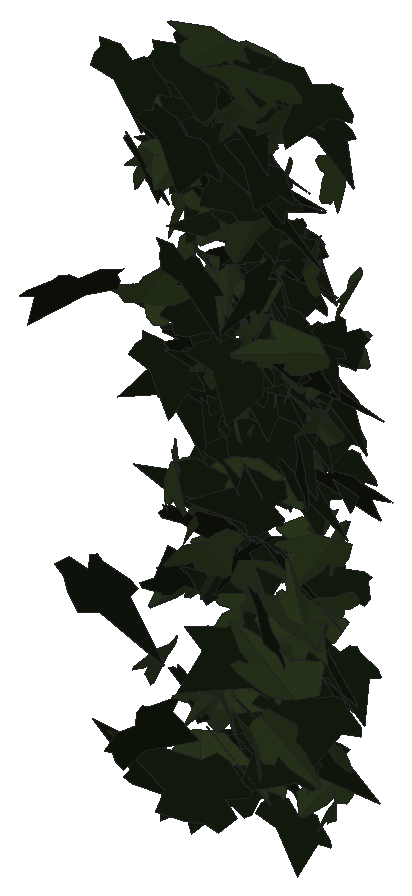
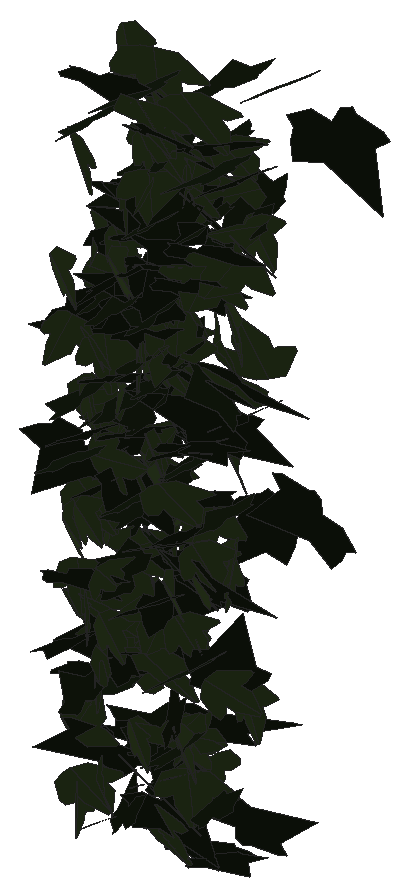
# SketchUp Ruby script. Lengths in millimetres.
U = 1.mm
M = Sketchup.active_model
def pt(a) = Geom::Point3d.new(a.map { |v| v * U })
def face(e, loops, mat)
  f = e.add_face(loops[0].map { |a| pt(a) })
  loops[1..].each { |l| e.add_face(l.map { |a| pt(a) }).erase! }
  f.material = f.back_material = mat if mat
  f
end
# faces: each face lists its corners as indices into pts; further lists are holes
def faces(e, pts, list, mat = nil) = list.each { |f| face(e, (f[0].is_a?(Array) ? f : [f]).map { |l| l.map { |i| pts[i] } }, mat) }
# xy, xz, yz: faces in a plane at the given z, y or x. An outline is a flat list of corners, or four numbers for a rectangle; further outlines are holes
def ring(l) = l.size == 4 ? [[l[0], l[1]], [l[2], l[1]], [l[2], l[3]], [l[0], l[3]]] : l.each_slice(2).to_a
def flat(e, list, mat, &to3) = list.each { |f| face(e, (f[0].is_a?(Array) ? f : [f]).map { |l| ring(l).map { |u, v| to3.(u, v) } }, mat) }
def xy(e, z, list, mat = nil) = flat(e, list, mat) { |x, y| [x, y, z] }
def xz(e, y, list, mat = nil) = flat(e, list, mat) { |x, z| [x, y, z] }
def yz(e, x, list, mat = nil) = flat(e, list, mat) { |y, z| [x, y, z] }
def lines(e, pts, list) = list.each { |a, b| e.add_line(pt(pts[a]), pt(pts[b])) }
# prism: a flat outline (further loops are holes) pulled along v
def prism(e, loops, v, mat = nil)
  f = face(e, loops, mat); d = Geom::Vector3d.new(v.map { |x| x * U })
  f.pushpull(f.normal.samedirection?(d) ? d.length : -d.length)
end
def box(e, o, s, mat = nil) = prism(e, [[o, [o[0] + s[0], o[1], o[2]], [o[0] + s[0], o[1] + s[1], o[2]], [o[0], o[1] + s[1], o[2]]]], [0, 0, s[2]], mat)
def at(x, y, z, deg = 0) = Geom::Transformation.translation(pt([x, y, z])) * Geom::Transformation.rotation(ORIGIN, Z_AXIS, deg.degrees)
def axes(o, x, y, z) = Geom::Transformation.new([*x, 0, *y, 0, *z, 0, *pt(o).to_a, 1])
def part(name) = M.definitions.add(name)
# library, detail: a bought-in or finely detailed component or shape, given as its bounding box
def library(name, o, s) = part(name).tap { |d| box(d.entities, o, s) }
def detail(e, o, s) = box(e.add_group.entities, o, s)
def put(e, d, t, mat = nil) = e.add_instance(d, t).tap { |i| i.material = mat if mat }
def group(e, t, mat = nil) = e.add_group.tap { |g| g.transformation = t; g.material = mat if mat }.entities
root = M.entities
M.materials.add("efeu1").color = [18, 25, 13]
M.materials.add("efeu2").color = [43, 57, 29]
c1 = part("ivyleaf_10")
p = [[0,12.8,-0.8],[-1.5,51.3,-10.9],[-4.9,51,-11.6],[-13.6,26.5,-7.3],[-13.2,15.9,-4.6],[-21.1,19.3,-7.2],
  [-29.5,16.3,-8.3],[-29.2,8.3,-6.2],[-19.7,-9.8,0.5],[-7.6,-13,4],[1,-12.2,5.8],[-0.4,51.1,-11.1],
  [-1.5,51.1,-10.9],[1,-12.4,5.9],[16.9,-12.4,3.5],[35.1,9.1,-5.1],[35,12.9,-6.1],[20.5,16.4,-4.9],
  [15.8,15,-3.8],[15.3,27.6,-7.1],[12.8,31.3,-7.8]]
faces(c1.entities,p,[[0,1,2,3,4,5,6,7,8,9,10],[11,12,0,13,14,15,16,17,18,19,20]],"efeu2")
c2 = part("ivyleaf_9")
p = [[39.1,54.8,31.7],[34.5,51.8,30.2],[-5.3,25.2,17.3],[-17.9,28.3,20.9],[-21.6,21.7,17],[-20.2,4.3,5.3],
  [-22.9,-0.3,2.5],[-17.1,-4,-0.6],[-2,-2.1,-1.2],[-0.7,-15.4,-10.1],[16.6,-22.3,-16.7],[21.1,-15.1,-12.5],
  [32.7,-10.7,-11],[46.1,-1.8,-6.6],[30.8,11.2,3.8]]
faces(c2.entities,p,[[0,1,2,3,4,5,6,7,8,9,10,11,12,13,14]],"efeu1")
put(root,c1,axes([2370.1,876.6,2356.8],[0.60294,-0.8909,-0.24909],[-0.05038,0.25445,-0.94375],[1.75987,0.31251,0.05832]))
put(root,c1,axes([2378.9,889.4,1882.8],[-0.34168,-0.62629,0.72512],[-0.30507,-0.70771,-0.65094],[1.79784,-0.23911,0.02736]))
put(root,c1,axes([2372.9,830.5,2450.6],[-0.06453,-0.98735,0.19467],[0.00299,-0.19483,-0.9879],[1.9153,-0.03296,0.0081]))
put(root,c1,axes([2354.5,855.3,2466.6],[0.48026,0.03585,-1.00007],[0.86211,0.91557,0.14712],[1.69827,-0.47492,0.20813]))
put(root,c1,axes([2363.1,882.7,2430.9],[-1.63571,-0.35297,-0.36931],[0.67826,0.10361,-0.92839],[0.69661,-0.92969,0.03675]))
put(root,c2,axes([2408.1,817,1664.1],[0.1409,-0.06142,0.97578],[-1.59712,0.49814,0.09503],[-0.95482,-0.8423,-0.01495]))
put(root,c1,axes([2390.6,853.3,2039.9],[-0.88376,0.56277,0.68264],[-0.77206,0.54969,-0.72911],[-1.49633,-0.616,-0.02698]))
put(root,c1,axes([2373,822.3,2270.3],[-1.0554,-0.86595,0.15564],[0.17943,0.12443,1.02822],[-1.66484,0.56237,0.01215]))
put(root,c2,axes([2363.9,893.8,2108.3],[0.13845,-0.89281,0.30246],[0.11131,-0.2985,-0.89519],[1.7906,0.08759,0.03226]))
put(root,c1,axes([2385.4,858.4,2023.6],[0.17024,-0.72433,-0.6179],[0.02917,0.62164,-0.72649],[1.81176,0.05805,0.06976]))
put(root,c2,axes([2381.9,870.7,1884],[1.11058,0.35379,0.7817],[-1.27053,-0.40669,0.68241],[1.0259,-0.88666,-0.00109]))
put(root,c2,axes([2423,854.5,2254.5],[-1.28585,0.28963,0.67405],[-1.2505,0.16875,-0.73109],[-0.62112,-0.93933,0.07649]))
put(root,c2,axes([2375.3,903.8,1728.1],[-0.29406,-0.50177,0.73344],[0.1244,-0.74884,-0.49854],[1.68671,-0.03225,0.16464]))
put(root,c2,axes([2379.1,873.8,2522.8],[-0.482,-1.00816,0.31724],[-0.09348,-0.31464,-1.03912],[2.00932,-0.25648,0.02776]))
put(root,c2,axes([2397,899.2,2443],[-1.52442,-0.55514,-0.05475],[0.07746,0.03739,-0.97452],[1.05883,-0.80198,-0.00753]))
put(root,c2,axes([2366.7,884.4,2553.1],[1.03738,-0.70362,-0.44634],[-0.0856,0.50774,-0.85532],[1.58352,0.48839,0.24617]))
put(root,c1,axes([2400,811.6,1832.3],[-0.14533,-1.02546,-0.052],[0.01465,0.05157,-1.02829],[1.95411,-0.07665,0.00384]))
put(root,c2,axes([2400.1,869.9,1647.9],[-1.02548,-0.65567,0.16211],[-0.19677,-0.12486,-0.84866],[1.27029,-0.54865,-0.00059]))
put(root,c2,axes([2379.3,847.4,2447.7],[-0.26472,-0.58411,0.79595],[0.32621,-0.80589,-0.56145],[1.85046,0.05851,0.21284]))
put(root,c2,axes([2402.8,863.3,2248.3],[-0.81059,0.70136,-0.55817],[-0.54532,0.47903,0.82055],[1.61645,0.51331,-0.00308]))
put(root,c2,axes([2436.5,875.5,2002],[-0.9212,0.32589,0.79539],[-1.26454,0.43727,-0.58349],[-1.03788,-0.82203,0.00495]))
put(root,c2,axes([2432.5,857.6,2462.2],[-1.28128,0.63694,0.39748],[-0.57904,0.25662,-0.92654],[-1.30631,-0.73848,0.02084]))
put(root,c2,axes([2419.3,844.5,2184.2],[0.03667,0.08127,-0.98957],[-0.31616,-0.97554,-0.08335],[-1.86306,0.16715,-0.00533]))
put(root,c1,axes([2409,885.2,2041.3],[-0.68455,-0.80088,0.33456],[-0.06296,-0.34924,-0.87158],[1.65068,-0.34545,0.1055]))
put(root,c2,axes([2389.9,767.7,2596.8],[-0.22027,-1.00161,0.18712],[0.0791,-0.19281,-1.00635],[1.93764,-0.10599,0.06236]))
put(root,c1,axes([2384.5,875.7,2318.5],[0.75735,-0.4455,0.75595],[1.05987,-0.51324,-0.59561],[1.29055,0.68294,0.04552]))
put(root,c2,axes([2386.3,795.6,2454],[0.0325,-0.53645,0.8538],[0.15085,-0.85056,-0.536],[1.91314,0.07618,0.02776]))
put(root,c2,axes([2410.8,903.9,2189.6],[-1.28106,-0.67117,0.11029],[-0.03843,-0.13538,-0.94708],[1.29393,-0.66851,0.08107]))
put(root,c2,axes([2396.5,828.5,2196.8],[-0.32281,-0.91761,0.26402],[-0.04634,-0.26391,-0.93287],[1.81666,-0.16979,0.02312]))
put(root,c1,axes([2383.4,852.6,2254.7],[1.36393,0.48313,0.53213],[0.81614,0.31563,-0.86409],[-1.09775,0.83494,0.01874]))
put(root,c1,axes([2404.8,881.6,2399.2],[-1.85741,-0.06903,-0.18062],[0.35835,-0.12778,-0.96854],[0.08375,-0.98425,0.13841]))
put(root,c2,axes([2419.8,895.2,2389.5],[-1.46161,-0.59788,-0.03979],[0.07548,0.01383,-0.97317],[1.1379,-0.76888,0.01344]))
put(root,c2,axes([2400.8,862.8,2560.5],[-0.50789,-0.97619,-0.13817],[0.35208,0.09102,-1.00037],[1.84307,-0.28639,0.15302]))
put(root,c1,axes([2422.9,887.2,1747.1],[-1.36173,-0.68219,0.02217],[-0.01371,-0.02457,-0.98851],[1.29896,-0.71542,0.01281]))
put(root,c1,axes([2440.6,864,2597.2],[-1.51766,-0.30381,0.53872],[-0.87491,-0.29688,-0.8479],[0.78744,-0.9154,0.09619]))
put(root,c2,axes([2397.9,885.3,1909.1],[0.9495,-0.68449,-0.52478],[-0.19715,0.55431,-0.82148],[1.62965,0.46587,0.20638]))
put(root,c1,axes([2420.9,866.9,2004.6],[0.34769,-0.89521,0.50998],[0.14021,-0.50526,-0.91332],[1.95582,0.19537,-0.02519]))
put(root,c2,axes([2392.4,859.8,2417],[1.28778,-0.73378,0.06745],[0.11879,-0.03417,-0.99788],[1.39739,0.67913,0.02267]))
put(root,c1,axes([2427.5,893.9,1946.6],[-0.53298,-0.81154,0.37848],[0.03931,-0.4023,-0.84734],[1.70377,-0.24459,0.13795]))
put(root,c2,axes([2423.1,863.3,1654.2],[-1.09817,-0.63215,-0.13567],[0.20354,0.08602,-0.85565],[1.21356,-0.58647,0.02074]))
put(root,c2,axes([2389,860.8,2202.9],[0.92031,0.58951,-0.63295],[0.75243,0.49433,0.76244],[1.46416,-0.62458,0.00603]))
put(root,c1,axes([2429.5,893.6,1801.9],[0.52448,-0.90268,-0.01144],[-0.00668,0.01089,-0.94381],[1.71811,0.2756,-0.00018]))
put(root,c1,axes([2442.5,902.7,2116.1],[-1.14985,-0.50426,0.53331],[-0.31399,-0.57978,-0.73509],[1.36114,-0.55973,0.28096]))
put(root,c2,axes([2419.9,842.8,1995.5],[1.74597,0.37331,-0.16882],[-0.305,-0.05405,-0.99038],[-0.71764,0.93122,0.0102]))
put(root,c2,axes([2424.6,868.1,2253.8],[-1.3374,-0.47324,-0.42634],[0.91672,0.02059,-0.81676],[0.79324,-0.82167,0.22509]))
put(root,c2,axes([2412.3,869.1,2457.6],[0.42749,-0.96117,0.10089],[0.045,-0.09808,-0.98707],[1.8388,0.22586,0.0007]))
put(root,c1,axes([2436.7,857.7,1929.6],[0.41171,-0.90661,-0.06868],[-0.03677,0.06599,-0.93206],[1.73002,0.21716,-0.00347]))
put(root,c2,axes([2431.6,896.5,2172.6],[-0.74147,-0.81672,0.31633],[-0.15059,-0.31198,-0.90293],[1.66008,-0.39308,0.05938]))
put(root,c1,axes([2415.8,794.2,2463.5],[-0.55187,-0.29863,-0.92444],[1.37736,0.57719,-0.41346],[1.23344,-0.77815,0.04809]))
put(root,c1,axes([2438.8,857.4,2391.2],[1.59977,-0.56842,-0.03707],[-0.05699,0.02189,-1.01471],[1.08261,0.8411,0.00136]))
put(root,c2,axes([2423.4,896.4,1792.9],[0.65775,-0.8414,-0.15455],[-0.08957,0.14773,-0.90953],[1.62568,0.34857,0.01242]))
put(root,c2,axes([2430.1,881.2,2063.2],[-0.04005,-0.94215,-0.15196],[-0.02947,0.15231,-0.94221],[1.81604,-0.01831,-0.01864]))
put(root,c1,axes([2449.6,782.6,2501.4],[-0.64489,-0.75966,0.57853],[0.05006,-0.62106,-0.80011],[1.81661,-0.25256,0.22742]))
put(root,c2,axes([2439,874.6,2136.9],[-0.53402,-0.72294,0.61402],[-0.16457,-0.61816,-0.76733],[1.79767,-0.27135,0.11215]))
put(root,c1,axes([2442.1,848.8,1774.7],[0.17094,-0.36941,0.91137],[0.32869,-0.89501,-0.3798],[1.8425,0.19394,-0.0168]))
put(root,c1,axes([2444.5,844.4,2511.5],[-0.14851,-0.85517,-0.54167],[0.3167,0.52505,-0.85291],[1.90038,-0.15433,0.09981]))
put(root,c2,axes([2467.4,877,1698.4],[0.55428,0.30012,-0.82426],[-1.03877,-0.61791,-0.41783],[-1.30696,0.61839,-0.01748]))
put(root,c1,axes([2447.5,873,2292.8],[-1.68321,0.40098,0.244],[0.38733,-0.14143,0.97009],[0.80499,0.90648,0.04342]))
put(root,c1,axes([2451.1,860.6,1790],[0.14397,-0.88661,0.28067],[0.12251,-0.27593,-0.88899],[1.76569,0.09144,0.03879]))
put(root,c2,axes([2411.6,668.6,1996.4],[-0.34954,-0.06917,-1.25975],[2.36962,0.19576,-0.19227],[0.38798,-1.25793,0.03935]))
put(root,c1,axes([2457.3,848.5,2211.5],[-0.33332,-0.95781,0.01471],[-0.00451,-0.01452,-0.97369],[1.82312,-0.17515,0.00028]))
put(root,c2,axes([2469.5,570.7,2433.8],[-0.00876,1.10977,-0.65289],[0.03152,-0.65279,-1.10972],[-2.45032,-0.01237,-0.01194]))
put(root,c2,axes([2442.9,892.9,1807.3],[-0.10594,-0.10811,1.03495],[-0.20094,-1.03049,-0.11332],[1.97021,-0.11091,0.04409]))
put(root,c2,axes([2447.6,905,1748.1],[-0.56399,-0.78994,0.22667],[0.07678,-0.25465,-0.8347],[1.56219,-0.27267,0.12286]))
put(root,c1,axes([2450.3,849.6,1781.4],[-0.76826,0.89574,-0.10741],[0.0821,-0.09837,-0.98249],[-1.71501,-0.40596,0.00108]))
put(root,c1,axes([2452.4,815.8,1728],[0.94159,1.02493,-0.23982],[-0.26047,-0.20011,-1.13753],[-1.98632,0.51209,0.03548]))
put(root,c1,axes([2454.7,856.7,2483.9],[1.70628,-0.46798,-0.03156],[-0.05035,0.01753,-1.01132],[0.89126,0.89692,0.00329]))
put(root,c1,axes([2465.5,859.4,1771.5],[1.40393,0.6168,0.26162],[-0.40791,-0.15143,0.96134],[1.20813,-0.7679,0.02056]))
put(root,c2,axes([2492,876.3,2550.5],[-1.75832,0.19924,0.30531],[-0.60671,-0.03792,-0.93989],[-0.33666,-0.97228,0.09922]))
put(root,c1,axes([2457.3,875.7,1976.4],[0.67868,-0.77108,0.40331],[0.28882,-0.37408,-0.84937],[1.63076,0.38716,-0.01742]))
put(root,c1,axes([2465.1,873.8,2268.1],[-0.47014,-0.83242,0.43741],[0.09967,-0.46372,-0.85293],[1.78689,-0.19315,0.16266]))
put(root,c2,axes([2443,876.1,2288.3],[0.04433,-0.61386,0.74538],[0.31381,-0.73212,-0.60809],[1.81077,0.14191,0.08713]))
put(root,c1,axes([2471.8,862.2,2296.2],[-0.91599,-0.73926,0.36851],[-0.099,-0.39853,-0.86741],[1.56895,-0.45674,0.16041]))
put(root,c2,axes([2461.3,899.5,2040.2],[-0.89184,-0.73714,0.27454],[0.04279,-0.33198,-0.853],[1.49645,-0.42982,0.18801]))
put(root,c2,axes([2491.5,871.7,2376.4],[-1.51102,-0.03572,0.5529],[-0.91107,-0.44221,-0.71596],[0.53091,-0.86052,0.34498]))
put(root,c2,axes([2490,863.7,2021.9],[-1.39388,0.67531,-0.07106],[0.09594,-0.05015,-0.99621],[-1.28878,-0.73412,0.00269]))
put(root,c1,axes([2442.6,773.1,2091.7],[0.29635,-0.17233,1.06385],[1.42757,-0.75449,-0.232],[1.47279,0.766,0.01082]))
put(root,c2,axes([2482.9,845.6,1675.7],[-0.99663,-0.43526,0.55721],[-0.7856,-0.37476,-0.68067],[1.09254,-0.66652,0.01885]))
put(root,c2,axes([2475,880.6,1959.7],[-0.49922,0.56333,-0.71902],[0.60046,-0.64617,-0.62135],[-1.63143,-0.41021,-0.00867]))
put(root,c1,axes([2478.9,840.6,2030.5],[-0.2538,0.62433,-0.79285],[-0.26807,0.7804,0.63822],[1.90184,0.19332,-0.01585]))
put(root,c1,axes([2485.5,877.5,1879.9],[1.55099,-0.02544,-0.54891],[-1.04363,0.02554,-0.8153],[0.0673,0.98223,0.00698]))
put(root,c1,axes([2480.7,869.5,2544.1],[1.76072,-0.16992,-0.3926],[-0.67817,0.21151,-0.93122],[0.45052,0.98248,0.13257]))
put(root,c1,axes([2472.8,869.5,1937.6],[-1.63655,-0.44619,-0.22946],[0.38686,0.10646,-0.96877],[0.87303,-0.88359,-0.00086]))
put(root,c1,axes([2459.7,846.3,2329.8],[1.20864,-0.61955,0.52491],[0.75455,-0.34497,-0.88683],[1.34871,0.74821,0.02576]))
put(root,c1,axes([2491.7,875,1676.1],[1.37758,-0.35821,-0.59437],[-0.99099,0.28743,-0.80732],[0.87313,0.89139,0.02147]))
put(root,c2,axes([2459.2,828.2,2073.7],[-0.14388,-0.83801,-0.48407],[0.21253,0.47475,-0.83931],[1.82956,-0.12105,0.05943]))
put(root,c2,axes([2506.5,871.2,1718.1],[-0.94344,0.65477,0.44064],[-0.52997,0.34179,-0.82113],[-1.40547,-0.5684,0.01384]))
put(root,c2,axes([2437.5,881.8,2430.3],[1.02529,-0.32013,0.77885],[1.30041,-0.37422,-0.62642],[0.93669,0.86994,0.01714]))
put(root,c2,axes([2442.5,889.3,2461.5],[0.72975,-0.62183,0.667],[0.97291,-0.45261,-0.71583],[1.43719,0.62214,0.14591]))
put(root,c1,axes([2484,881.2,2492.3],[-1.20769,-0.76366,-0.01621],[0.06142,-0.00575,-0.99249],[1.45243,-0.63474,0.02849]))
put(root,c2,axes([2457.2,822.8,2510.6],[0.5906,-0.92507,-0.29054],[-0.01274,0.30301,-0.97191],[1.84535,0.29816,0.08628]))
put(root,c2,axes([2466.1,892.9,2452.3],[0.04121,-0.95056,0.25963],[0.06898,-0.25875,-0.95036],[1.87411,0.03043,0.02927]))
put(root,c1,axes([2488.7,881.1,2582.6],[1.76479,-0.20646,-0.31299],[-0.53447,0.1708,-0.94466],[0.47282,0.96365,0.10038]))
put(root,c2,axes([2464.3,882.6,2246],[0.26884,-0.91706,0.28445],[0.08917,-0.28059,-0.92787],[1.8252,0.14879,0.00343]))
put(root,c1,axes([2489.1,838,2546.5],[0.20982,-0.99371,0.21264],[0.01108,-0.21327,-0.99966],[1.93402,0.10903,-0.01734]))
put(root,c2,axes([2478.6,875.9,2298.3],[-0.84851,-0.80919,-0.30244],[0.24259,0.275,-0.92366],[1.62611,-0.46326,-0.02002]))
put(root,c2,axes([2491.5,855.9,2197.2],[-1.48583,0.30952,-0.54833],[0.98046,-0.18822,-0.83973],[-0.68904,-0.93527,-0.01247]))
put(root,c2,axes([2477.4,904.5,1958.8],[-0.39145,-0.87645,0.17192],[-0.02103,-0.1739,-0.89981],[1.69971,-0.204,0.02846]))
put(root,c2,axes([2499.6,851.9,2361.3],[0.33991,0.81012,-0.57667],[-0.25608,-0.56082,-0.82953],[-1.87515,0.22344,0.00875]))
put(root,c1,axes([2492.8,854.4,2579.8],[0.53914,-0.95506,-0.17778],[-0.06717,0.17494,-0.99606],[1.84767,0.28504,0.01566]))
put(root,c1,axes([2494.2,841,2553.4],[-0.08911,-1.03351,0.08589],[-0.02648,-0.08534,-1.03452],[1.97358,-0.04781,-0.01]))
put(root,c2,axes([2475.1,845.2,2098.1],[0.06269,-0.92582,0.25483],[0.00066,-0.25496,-0.92636],[1.82754,0.03185,-0.00841]))
put(root,c1,axes([2492.9,840.1,2143],[-0.05126,0.50115,0.88677],[-0.42895,0.86216,-0.49409],[-1.89052,-0.20921,0.08806]))
put(root,c2,axes([2470.7,865.7,2520.6],[0.17609,-0.90579,0.4396],[0.21133,-0.42958,-0.90851],[1.9045,0.13142,0.06016]))
put(root,c2,axes([2471.8,863.5,2093.5],[0.10785,-0.73281,0.71531],[0.24351,-0.70573,-0.73313],[1.9337,0.12975,0.05243]))
put(root,c1,axes([2488.7,878,2486.2],[-0.37835,0.92137,-0.36264],[-0.05965,-0.37555,-0.93698],[-1.88355,-0.17318,0.10251]))
put(root,c1,axes([2496.4,891.3,1787.5],[0.16245,-0.87572,0.01385],[0.00941,-0.01344,-0.87987],[1.66686,0.08542,0.00362]))
put(root,c2,axes([2491.4,846.4,2220.1],[-0.99057,-0.91662,0.05668],[-0.04113,-0.05291,-1.05405],[1.74735,-0.52087,0.00732]))
put(root,c2,axes([2534.2,744,1721.8],[-1.58514,-0.68543,-0.49251],[-0.68635,-0.33659,1.07829],[-1.45233,0.90717,0.02796]))
put(root,c2,axes([2513.3,826.7,1856.7],[-1.58752,-0.54906,0.36469],[-0.57916,-0.20099,-0.99862],[1.11279,-0.88791,0.00053]))
put(root,c1,axes([2493.8,772,2016.5],[-1.00725,-0.92173,-0.5177],[0.44737,0.46185,-1.0626],[1.96162,-0.57862,-0.02349]))
put(root,c2,axes([2473.6,883.4,2327.6],[0.50614,-0.9144,0.23622],[0.10527,-0.22991,-0.95223],[1.79434,0.27142,-0.01077]))
put(root,c1,axes([2500.7,861.5,2531.5],[-0.33969,-0.99942,-0.03547],[0.02199,0.03397,-1.01521],[1.90316,-0.17878,0.0054]))
put(root,c1,axes([2501.2,868.2,2170.5],[1.06122,-0.85436,-0.29665],[-0.23127,0.27456,-1.01917],[1.70564,0.5688,0.04638]))
put(root,c2,axes([2489.5,844.2,2476.6],[-0.88285,-0.85031,-0.28636],[0.21657,0.26401,-0.96828],[1.69383,-0.47695,-0.02546]))
put(root,c1,axes([2499.7,861.1,2263.8],[0.06919,-0.95414,0.32812],[0.10997,-0.32582,-0.95387],[1.91714,0.05312,0.04287]))
put(root,c1,axes([2495.9,864.5,2126.6],[0.50886,-0.74185,0.71446],[0.46273,-0.67182,-0.78856],[1.9048,0.36139,0.0007]))
put(root,c2,axes([2525.6,868.4,1862],[-1.27205,-0.13619,0.57994],[-0.89814,-0.4109,-0.64036],[0.69194,-0.78372,0.23496]))
put(root,c2,axes([2475.8,839.9,1707.4],[0.2395,-0.59106,0.85278],[0.55303,-0.80458,-0.60053],[1.89571,0.30939,0.06745]))
put(root,c2,axes([2490.4,736.1,2550.9],[-0.51477,-0.91346,0.63383],[0.11365,-0.66331,-0.93046],[2.11296,-0.18686,0.20446]))
put(root,c2,axes([2477.8,887.9,2204.9],[1.00525,-0.79931,0.11524],[0.09505,-0.1051,-0.95792],[1.53402,0.5303,-0.01616]))
put(root,c2,axes([2463.4,870.1,2345],[1.30508,-0.35834,0.64251],[1.09472,-0.28645,-0.77365],[0.87293,0.89498,0.00964]))
put(root,c2,axes([2463.2,824.6,2431.8],[0.89217,-0.01387,0.92012],[1.74718,-0.06435,-0.46868],[0.1211,1.03065,-0.01688]))
put(root,c1,axes([2509.2,834.8,1938.3],[0.4696,-0.86075,-0.33384],[-0.13153,0.32737,-0.89514],[1.75215,0.25527,0.02228]))
put(root,c2,axes([2506.6,895.8,2169],[-1.00481,-0.72287,0.34937],[-0.20025,-0.35224,-0.88781],[1.51485,-0.52605,0.11438]))
put(root,c2,axes([2482.8,894.3,2082.6],[0.74641,-0.87273,-0.02052],[-0.0172,0.01844,-0.9568],[1.66136,0.39229,-0.00069]))
put(root,c2,axes([2487.1,889.9,2263.4],[0.30737,-0.95761,0.10475],[0.01,-0.10534,-0.97106],[1.83338,0.16112,-0.01226]))
put(root,c1,axes([2509.5,840,2299.5],[1.00099,-0.89855,-0.15739],[-0.09585,0.1528,-1.04063],[1.73351,0.52731,0.03335]))
put(root,c2,axes([2495,860,2187.6],[-0.19903,-0.88782,0.3919],[0.19397,-0.40204,-0.88359],[1.83679,-0.05375,0.13578]))
put(root,c2,axes([2495.4,895.8,2084.5],[-0.07725,-0.89422,0.31066],[0.12818,-0.31289,-0.89182],[1.79709,-0.01612,0.07697]))
put(root,c2,axes([2524.4,865,2092],[-0.12545,0.73189,-0.68623],[0.09981,-0.68426,-0.73482],[-1.90683,-0.08397,0.00668]))
put(root,c1,axes([2512.3,862.6,2264.6],[0.61956,-0.81031,-0.47547],[0.11176,0.51977,-0.8456],[1.78458,0.24877,0.21803]))
put(root,c2,axes([2505.4,900.8,1674.5],[-0.35337,-0.17571,0.87269],[-0.16909,-0.88336,-0.19676],[1.68577,-0.12544,0.1632]))
put(root,c1,axes([2526.5,831,2092],[1.7144,0.23143,-0.43295],[-0.80852,-0.08596,-0.92983],[-0.46825,0.99574,0.02035]))
put(root,c1,axes([2531.2,815.5,2602.9],[-1.9133,-0.36923,0.13491],[-0.24459,-0.0414,-1.07095],[0.70705,-1.01347,-0.0054]))
put(root,c2,axes([2500,844.2,2596.8],[1.0916,-0.6952,-0.49424],[-0.15004,0.54983,-0.86488],[1.61644,0.52051,0.25349]))
put(root,c1,axes([2523.6,890.6,2375.4],[0.63592,-0.86401,0.32754],[0.16536,-0.31738,-0.92583],[1.75079,0.3438,-0.03153]))
put(root,c1,axes([2526.4,864.2,2459.3],[-0.02203,-0.92088,-0.36017],[0.13846,0.35843,-0.91875],[1.8768,-0.03725,0.06355]))
put(root,c2,axes([2521.8,853.8,2401.3],[-0.9164,-0.94792,0.18575],[-0.07115,-0.18911,-1.06195],[1.83701,-0.4802,0.05153]))
put(root,c2,axes([2496.2,854.7,1761.6],[0.44539,-0.66624,0.62095],[0.64772,-0.53071,-0.69768],[1.60777,0.39837,0.10905]))
put(root,c1,axes([2530.6,853,2096.1],[0.88135,-0.84092,-0.16179],[-0.12174,0.14945,-0.95987],[1.62524,0.46722,0.01584]))
put(root,c2,axes([2515.1,820.9,2458.5],[-0.60363,-0.84929,-0.49362],[0.33797,0.46059,-0.90657],[1.83874,-0.36347,0.00459]))
put(root,c1,axes([2538,856.6,2176.5],[0.39161,-0.34128,0.92237],[-0.8297,0.81305,0.39808],[-1.67782,-0.48172,0.01843]))
put(root,c2,axes([2534.3,896.1,2229.9],[-1.1199,-0.66178,0.34522],[-0.18007,-0.36992,-0.8704],[1.40912,-0.57323,0.16314]))
put(root,c1,axes([2559.2,870,2108.6],[-0.54583,0.26981,-0.92976],[-1.30856,0.62591,0.39372],[1.29714,0.74495,0.00594]))
put(root,c2,axes([2513.8,894.1,2197.1],[0.06949,-0.83414,0.48184],[0.08484,-0.4802,-0.83469],[1.8314,0.0539,0.02039]))
put(root,c2,axes([2564.1,794.6,2081],[-1.48479,0.55686,0.33471],[-0.54769,0.17277,-0.95818],[-1.10862,-0.83116,0.02508]))
put(root,c1,axes([2536.6,892.3,1910.6],[-0.10158,-0.87974,0.16389],[-0.03273,-0.16315,-0.88133],[1.70282,-0.05562,-0.00716]))
put(root,c2,axes([2515.4,890.3,2366.1],[0.48188,-0.84427,-0.44731],[-0.14696,0.44315,-0.88014],[1.81246,0.2604,0.04756]))
put(root,c1,axes([2539.9,788.4,2430.3],[-0.64605,-0.94471,0.07458],[-0.01964,-0.07553,-1.00372],[1.80346,-0.33924,0.01579]))
put(root,c2,axes([2524.5,838.4,2482.6],[-0.44309,-0.75278,0.62439],[-0.02954,-0.63891,-0.77607],[1.86115,-0.18936,0.13634]))
put(root,c1,axes([2530,907,1984.2],[-0.43936,-0.65604,0.68278],[0.48795,-0.71984,-0.60496],[1.73478,0.03632,0.34308]))
put(root,c1,axes([2545.7,798.7,2339.6],[1.21524,-0.64671,0.75688],[-0.99806,0.54582,0.90878],[-1.61053,-0.82623,0.00793]))
put(root,c2,axes([2527.9,895.9,2314.8],[-0.26503,-0.75943,0.57512],[-0.03453,-0.57901,-0.76896],[1.81271,-0.12206,0.06944]))
put(root,c2,axes([2528.3,842.5,2142.9],[-0.6006,-0.59418,-0.764],[0.61354,0.69317,-0.67225],[1.73685,-0.45033,-0.02672]))
put(root,c1,axes([2550.3,852.2,2385.9],[-0.28684,-0.95944,-0.00725],[0.00551,0.00688,-0.97121],[1.82606,-0.15073,0.00179]))
put(root,c1,axes([2550.8,875.8,1859.9],[-0.24943,-0.79523,0.61361],[0.06257,-0.62187,-0.79892],[1.91064,-0.08345,0.10627]))
put(root,c1,axes([2533.8,904.6,1711.7],[0.65349,-0.58295,0.65261],[0.77204,-0.51513,-0.67358],[1.47565,0.52767,0.0634]))
put(root,c2,axes([2560.7,852.6,2395.5],[-0.17616,-0.20905,-0.99796],[0.20672,-0.99838,0.19907],[-1.9295,-0.08788,0.11244]))
put(root,c2,axes([2564.6,836,1744.4],[-1.38547,-0.48473,0.1836],[-0.29803,-0.09608,-0.87456],[0.9404,-0.74459,-0.00667]))
put(root,c2,axes([2525,866.2,1967.4],[0.9741,-0.81434,0.35155],[0.35663,-0.29745,-0.96183],[1.65,0.54504,0.00035]))
put(root,c2,axes([2543.3,886.3,1818.1],[-0.34847,-0.76964,0.39862],[0.23751,-0.42659,-0.76631],[1.63241,-0.10223,0.19659]))
put(root,c2,axes([2531.3,826.8,2445.5],[1.24148,-0.79787,-0.07517],[-0.07885,0.06322,-1.03056],[1.5232,0.65358,0.00792]))
put(root,c1,axes([2558.9,881,1840.6],[0.69293,-0.63901,-0.50636],[-0.02079,0.55068,-0.7028],[1.55156,0.29276,0.21672]))
put(root,c2,axes([2546.6,865.5,1648.9],[-0.3494,-0.88441,0.2176],[0.03298,-0.22533,-0.9012],[1.73309,-0.17401,0.06102]))
put(root,c1,axes([2564.8,857.1,2241.9],[-1.09492,-0.8316,-0.02307],[0.04056,0.01331,-1.01115],[1.58278,-0.57561,0.00995]))
put(root,c2,axes([2536.2,683,2429.7],[0.381,-1.06234,0.2828],[0.12734,-0.27514,-1.08094],[2.08838,0.21059,0.01432]))
put(root,c1,axes([2590.4,855.8,2159.8],[-1.12125,0.23193,-0.79402],[-1.40736,0.28923,0.63314],[0.70558,0.94546,0.00109]))
put(root,c2,axes([2547.7,877.5,2082.3],[-0.08705,-0.96219,0.00085],[-0.00162,-0.00081,-0.96327],[1.83124,-0.04574,-0.00081]))
put(root,c2,axes([2561.4,563.8,1900],[-0.08486,0.05768,-1.30468],[-0.90877,1.21433,0.07001],[2.3134,0.47914,-0.02036]))
put(root,c2,axes([2547.1,869.3,2176.1],[0.40026,-0.94092,0.02725],[-0.0014,-0.02808,-0.96411],[1.79151,0.2102,-0.00684]))
put(root,c1,axes([2557.1,830.2,1936.8],[-1.85393,-0.16567,-0.41792],[0.7941,0.03812,-0.98765],[0.31853,-1.05929,0.02982]))
put(root,c2,axes([2569.4,861,2588.9],[-1.50258,-0.5602,-0.24577],[0.43066,0.10537,-0.96708],[1.0817,-0.82013,0.04363]))
put(root,c1,axes([2580.2,886.2,1695.2],[-0.88984,-0.68496,0.55005],[-0.20723,-0.57311,-0.80624],[1.65903,-0.43898,0.19432]))
put(root,c2,axes([2584,898.7,1961.4],[-1.40551,-0.51051,0.1413],[-0.19824,-0.09774,-0.89753],[0.98845,-0.74552,0.02091]))
put(root,c2,axes([2566.3,905.7,2149.5],[-0.5134,-0.86744,0.2219],[-0.02833,-0.22738,-0.90694],[1.70384,-0.26516,0.05178]))
put(root,c2,axes([2541.5,874.5,1873.7],[-0.1125,-0.05941,-1.00876],[1.91075,0.11137,-0.06539],[0.21854,-1.00434,0.05242]))
put(root,c2,axes([2584.5,762,2388.9],[-1.41885,0.61879,-0.64215],[0.94587,-0.40666,-0.96885],[-1.40921,-0.89597,-0.00375]))
put(root,c1,axes([2541.7,851.3,1882.9],[1.25848,0.12602,-0.83],[1.55801,0.13745,0.67305],[0.35423,-1.05226,-0.01149]))
put(root,c1,axes([2580.3,880.2,2032.6],[0.19381,-0.85814,0.37338],[0.15658,-0.36593,-0.86343],[1.77421,0.12603,0.03542]))
put(root,c1,axes([2591.7,833.5,2374.2],[-0.09216,0.23077,1.02772],[-0.90226,0.91394,-0.22756],[-1.79014,-0.47252,0.06178]))
put(root,c2,axes([2560.2,904.1,1812.1],[0.28998,-0.6407,0.59543],[0.23777,-0.58226,-0.6585],[1.64759,0.1968,-0.00977]))
put(root,c2,axes([2559.7,846.5,2101.3],[0.98097,-0.79421,-0.18502],[-0.15159,0.1688,-0.94648],[1.54459,0.52097,0.02462]))
put(root,c1,axes([2584.4,880.6,1670.8],[0.15407,-0.74044,-0.52048],[0.06028,0.52455,-0.74131],[1.72147,0.0479,0.07254]))
put(root,c1,axes([2587.1,859.5,2178.2],[-0.01857,-0.98445,-0.19542],[0.02486,0.19528,-0.98444],[1.91,-0.01211,0.01091]))
put(root,c2,axes([2554.9,864.7,1740.1],[-0.0364,-0.18121,-0.89416],[1.23535,0.62578,-0.1407],[1.22018,-0.63897,0.11578]))
put(root,c1,axes([2614,797.4,2293.5],[-0.40548,-0.21782,1.03343],[-1.2646,-0.79181,-0.30388],[1.56238,-0.69742,0.02224]))
put(root,c2,axes([2566.1,882.1,2542.4],[0.33289,-0.98607,0.00592],[0.0388,-0.0024,-1.00126],[1.87631,0.17499,0.01965]))
put(root,c1,axes([2599.1,862.9,1747],[-1.63935,0.52009,-0.1853],[-0.30315,0.09469,1.0062],[1.00611,0.87597,0.00125]))
put(root,c1,axes([2589,862.5,1911.7],[0.45035,-0.82911,-0.36898],[0.09211,0.3923,-0.85048],[1.7247,0.19554,0.14176]))
put(root,c1,axes([2592.8,784.4,2598.5],[-0.01008,-1.04896,-0.16508],[0.04658,0.16491,-1.04871],[2.02041,-0.00904,0.02335]))
put(root,c2,axes([2568.4,898.4,2192.4],[0.49091,-0.92257,0.11035],[0.05067,-0.10714,-0.95795],[1.76763,0.25929,-0.00318]))
put(root,c2,axes([2582.4,833.3,2106.7],[-0.09891,0.02956,1.02328],[-0.37931,-1.00528,0.01892],[1.91103,-0.198,0.05672]))
put(root,c1,axes([2592.5,859.6,2247.3],[1.26226,-0.85002,-0.04538],[-0.04368,0.03965,-1.07813],[1.61946,0.6636,0.00629]))
put(root,c2,axes([2588.8,843.2,1818.6],[-1.00439,-0.91325,-0.1621],[0.17483,0.13412,-1.0547],[1.75659,-0.53553,0.01229]))
put(root,c2,axes([2580.9,901.9,2108],[-0.22304,-0.88757,0.32642],[0.191,-0.33873,-0.88502],[1.78968,-0.07447,0.13513]))
put(root,c1,axes([2587.4,737.8,1800.4],[-1.26808,0.74058,0.66765],[0.83193,-0.50477,0.99614],[1.70562,0.79681,0.01051]))
put(root,c1,axes([2601.7,860.2,1943.6],[-0.83354,-0.82794,-0.1091],[0.06897,0.10423,-0.9365],[1.58786,-0.43915,-0.01659]))
put(root,c2,axes([2561,825.7,2247],[1.62705,-0.2956,0.49709],[0.89239,-0.16507,-0.90456],[0.64434,0.97505,-0.00243]))
put(root,c1,axes([2592.8,888.7,2017.5],[0.69418,-0.7031,0.53576],[0.4943,-0.46875,-0.79198],[1.6081,0.4476,0.01217]))
put(root,c1,axes([2586.1,783.8,1904.4],[1.28546,-0.57706,0.4926],[0.70848,-0.32263,-0.88836],[1.25825,0.77121,-0.00305]))
put(root,c2,axes([2583.3,846.1,2290.8],[0.24974,-0.95878,0.22938],[0.1182,-0.2229,-0.96724],[1.87252,0.14194,0.03046]))
put(root,c1,axes([2613.8,832.3,2029.2],[-0.87937,-0.87705,0.45616],[-0.19856,-0.45745,-0.98521],[1.87097,-0.46077,0.10984]))
put(root,c1,axes([2608.3,856.7,2488.5],[1.01726,-0.76051,-0.38517],[-0.22677,0.38351,-0.92257],[1.60652,0.53569,0.11367]))
put(root,c1,axes([2611.3,786.1,1968.6],[-0.1662,0.91825,-0.43017],[-0.15297,0.42414,0.92169],[1.92381,0.11305,0.03612]))
put(root,c1,axes([2611.2,885.5,2342.8],[0.41967,-0.95136,0.0916],[0.01738,-0.0919,-0.97651],[1.81892,0.22038,-0.0118]))
put(root,c1,axes([2604.7,875.6,2264.2],[-0.65219,-0.71439,-0.57467],[0.51202,0.50815,-0.79211],[1.66812,-0.43528,0.01845]))
put(root,c2,axes([2610.4,870,2282.9],[-0.0369,0.10838,-1.01391],[0.72486,-0.93992,-0.10776],[-1.8002,-0.38069,-0.02261]))
put(root,c1,axes([2631.7,736.4,1905],[1.8077,0.14067,0.72978],[-1.36433,-0.13914,0.95983],[0.3733,-1.1897,-0.02597]))
put(root,c1,axes([2571.8,785.2,1801.5],[0.91092,-0.17826,1.05613],[1.96164,-0.2379,-0.50726],[0.55431,1.13485,0.05955]))
put(root,c2,axes([2597.7,879.3,1864.8],[-0.11736,-0.91246,-0.19558],[0.0843,0.19293,-0.91403],[1.77403,-0.06953,0.03049]))
put(root,c2,axes([2599,859.7,2103.2],[1.78425,0.21083,-0.15179],[-0.28644,-0.0225,-0.96085],[-0.403,0.94944,0.01094]))
put(root,c2,axes([2602,747.5,1960.4],[-0.24784,-0.2604,1.11383],[-0.1665,-1.11547,-0.27101],[2.17062,-0.1153,0.10639]))
